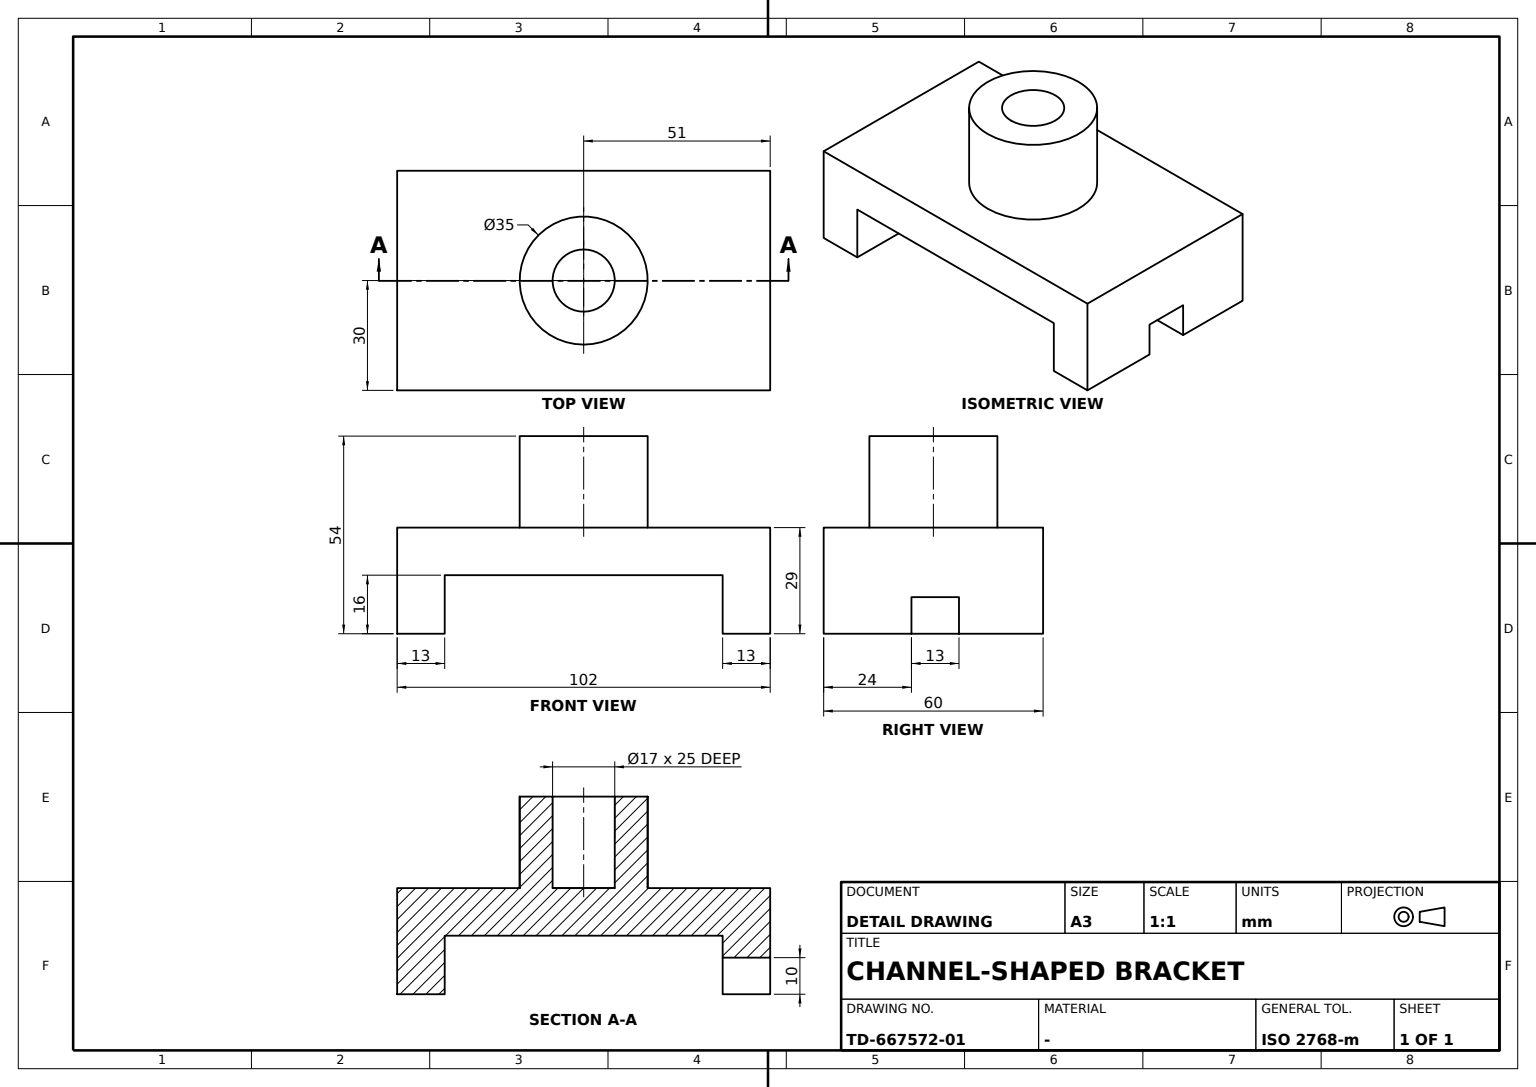
ISO-10303-21;
HEADER;
FILE_DESCRIPTION((''),'2;1');
FILE_NAME('','',(''),(''),'','','');
FILE_SCHEMA(('AUTOMOTIVE_DESIGN'));
ENDSEC;
DATA;
#1=APPLICATION_CONTEXT('');
#2=PRODUCT_CONTEXT('',#1,'mechanical');
#3=PRODUCT('','','',(#2));
#4=PRODUCT_DEFINITION_FORMATION('','',#3);
#5=PRODUCT_DEFINITION_CONTEXT('',#1,'design');
#6=PRODUCT_DEFINITION('','',#4,#5);
#7=PRODUCT_DEFINITION_SHAPE('','',#6);
#8=(LENGTH_UNIT()NAMED_UNIT(*)SI_UNIT(.MILLI.,.METRE.));
#9=(NAMED_UNIT(*)PLANE_ANGLE_UNIT()SI_UNIT($,.RADIAN.));
#10=(NAMED_UNIT(*)SI_UNIT($,.STERADIAN.)SOLID_ANGLE_UNIT());
#11=UNCERTAINTY_MEASURE_WITH_UNIT(LENGTH_MEASURE(0.005),#8,'distance_accuracy_value','');
#12=(GEOMETRIC_REPRESENTATION_CONTEXT(3)GLOBAL_UNCERTAINTY_ASSIGNED_CONTEXT((#11))GLOBAL_UNIT_ASSIGNED_CONTEXT((#8,#9,#10))REPRESENTATION_CONTEXT('',''));
#13=CARTESIAN_POINT('',(0.,38.,-29.));
#14=VERTEX_POINT('',#13);
#15=CARTESIAN_POINT('',(0.,38.,-13.));
#16=VERTEX_POINT('',#15);
#17=DIRECTION('',(0.,0.,1.));
#18=VECTOR('',#17,1000.);
#19=LINE('',#13,#18);
#20=EDGE_CURVE('',#14,#16,#19,.T.);
#21=ORIENTED_EDGE('',*,*,#20,.T.);
#22=CARTESIAN_POINT('',(-60.,38.,-13.));
#23=VERTEX_POINT('',#22);
#24=DIRECTION('',(-1.,0.,0.));
#25=VECTOR('',#24,1000.);
#26=LINE('',#15,#25);
#27=EDGE_CURVE('',#16,#23,#26,.T.);
#28=ORIENTED_EDGE('',*,*,#27,.T.);
#29=CARTESIAN_POINT('',(-60.,38.,-29.));
#30=VERTEX_POINT('',#29);
#31=LINE('',#29,#18);
#32=EDGE_CURVE('',#30,#23,#31,.T.);
#33=ORIENTED_EDGE('',*,*,#32,.F.);
#34=CARTESIAN_POINT('',(-37.,38.,-29.));
#35=VERTEX_POINT('',#34);
#36=LINE('',#13,#25);
#37=EDGE_CURVE('',#35,#30,#36,.T.);
#38=ORIENTED_EDGE('',*,*,#37,.F.);
#39=CARTESIAN_POINT('',(-37.,38.,-19.));
#40=VERTEX_POINT('',#39);
#41=DIRECTION('',(0.,0.,-1.));
#42=VECTOR('',#41,1000.);
#43=LINE('',#34,#42);
#44=EDGE_CURVE('',#40,#35,#43,.T.);
#45=ORIENTED_EDGE('',*,*,#44,.F.);
#46=CARTESIAN_POINT('',(-24.,38.,-19.));
#47=VERTEX_POINT('',#46);
#48=CARTESIAN_POINT('',(0.,38.,-19.));
#49=LINE('',#48,#25);
#50=EDGE_CURVE('',#47,#40,#49,.T.);
#51=ORIENTED_EDGE('',*,*,#50,.F.);
#52=CARTESIAN_POINT('',(-24.,38.,-29.));
#53=VERTEX_POINT('',#52);
#54=LINE('',#52,#18);
#55=EDGE_CURVE('',#53,#47,#54,.T.);
#56=ORIENTED_EDGE('',*,*,#55,.F.);
#57=EDGE_CURVE('',#14,#53,#36,.T.);
#58=ORIENTED_EDGE('',*,*,#57,.F.);
#59=EDGE_LOOP('',(#21,#28,#33,#38,#45,#51,#56,#58));
#60=FACE_BOUND('',#59,.T.);
#61=DIRECTION('',(0.,-1.,0.));
#62=AXIS2_PLACEMENT_3D('',#13,#61,#17);
#63=PLANE('',#62);
#64=ADVANCED_FACE('',(#60),#63,.T.);
#65=CARTESIAN_POINT('',(-37.,51.,-29.));
#66=VERTEX_POINT('',#65);
#67=CARTESIAN_POINT('',(-60.,51.,-29.));
#68=VERTEX_POINT('',#67);
#69=CARTESIAN_POINT('',(0.,51.,-29.));
#70=LINE('',#69,#25);
#71=EDGE_CURVE('',#66,#68,#70,.T.);
#72=ORIENTED_EDGE('',*,*,#71,.F.);
#73=VECTOR('',#61,1000.);
#74=LINE('',#65,#73);
#75=EDGE_CURVE('',#66,#35,#74,.T.);
#76=ORIENTED_EDGE('',*,*,#75,.T.);
#77=ORIENTED_EDGE('',*,*,#37,.T.);
#78=CARTESIAN_POINT('',(-60.,-38.,-29.));
#79=LINE('',#78,#73);
#80=EDGE_CURVE('',#68,#30,#79,.T.);
#81=ORIENTED_EDGE('',*,*,#80,.F.);
#82=EDGE_LOOP('',(#72,#76,#77,#81));
#83=FACE_BOUND('',#82,.T.);
#84=CARTESIAN_POINT('',(0.,-38.,-29.));
#85=AXIS2_PLACEMENT_3D('',#84,#41,#61);
#86=PLANE('',#85);
#87=ADVANCED_FACE('',(#83),#86,.T.);
#88=ORIENTED_EDGE('',*,*,#57,.T.);
#89=CARTESIAN_POINT('',(-24.,51.,-29.));
#90=VERTEX_POINT('',#89);
#91=CARTESIAN_POINT('',(-24.,-38.,-29.));
#92=LINE('',#91,#73);
#93=EDGE_CURVE('',#90,#53,#92,.T.);
#94=ORIENTED_EDGE('',*,*,#93,.F.);
#95=VERTEX_POINT('',#69);
#96=EDGE_CURVE('',#95,#90,#70,.T.);
#97=ORIENTED_EDGE('',*,*,#96,.F.);
#98=LINE('',#84,#73);
#99=EDGE_CURVE('',#95,#14,#98,.T.);
#100=ORIENTED_EDGE('',*,*,#99,.T.);
#101=EDGE_LOOP('',(#88,#94,#97,#100));
#102=FACE_BOUND('',#101,.T.);
#103=ADVANCED_FACE('',(#102),#86,.T.);
#104=ORIENTED_EDGE('',*,*,#55,.T.);
#105=CARTESIAN_POINT('',(-24.,51.,-19.));
#106=VERTEX_POINT('',#105);
#107=LINE('',#105,#73);
#108=EDGE_CURVE('',#106,#47,#107,.T.);
#109=ORIENTED_EDGE('',*,*,#108,.F.);
#110=LINE('',#89,#18);
#111=EDGE_CURVE('',#90,#106,#110,.T.);
#112=ORIENTED_EDGE('',*,*,#111,.F.);
#113=ORIENTED_EDGE('',*,*,#93,.T.);
#114=EDGE_LOOP('',(#104,#109,#112,#113));
#115=FACE_BOUND('',#114,.T.);
#116=DIRECTION('',(1.,0.,0.));
#117=AXIS2_PLACEMENT_3D('',#89,#116,#17);
#118=PLANE('',#117);
#119=ADVANCED_FACE('',(#115),#118,.F.);
#120=CARTESIAN_POINT('',(-21.5,0.,0.));
#121=VERTEX_POINT('',#120);
#122=CARTESIAN_POINT('',(-30.,0.,0.));
#123=AXIS2_PLACEMENT_3D('',#122,#17,#116);
#124=CIRCLE('',#123,8.5);
#125=EDGE_CURVE('',#121,#121,#124,.T.);
#126=ORIENTED_EDGE('',*,*,#125,.F.);
#127=EDGE_LOOP('',(#126));
#128=FACE_BOUND('',#127,.T.);
#129=CARTESIAN_POINT('',(-21.5,0.,25.));
#130=VERTEX_POINT('',#129);
#131=CARTESIAN_POINT('',(-30.,0.,25.));
#132=AXIS2_PLACEMENT_3D('',#131,#17,#116);
#133=CIRCLE('',#132,8.5);
#134=EDGE_CURVE('',#130,#130,#133,.T.);
#135=ORIENTED_EDGE('',*,*,#134,.T.);
#136=EDGE_LOOP('',(#135));
#137=FACE_BOUND('',#136,.T.);
#138=CARTESIAN_POINT('',(-30.,0.,12.5));
#139=AXIS2_PLACEMENT_3D('',#138,#17,#116);
#140=CYLINDRICAL_SURFACE('',#139,8.5);
#141=ADVANCED_FACE('',(#128,#137),#140,.F.);
#142=CARTESIAN_POINT('',(0.,-51.,-29.));
#143=VERTEX_POINT('',#142);
#144=CARTESIAN_POINT('',(0.,-51.,0.));
#145=VERTEX_POINT('',#144);
#146=LINE('',#142,#18);
#147=EDGE_CURVE('',#143,#145,#146,.T.);
#148=ORIENTED_EDGE('',*,*,#147,.T.);
#149=CARTESIAN_POINT('',(-60.,-51.,0.));
#150=VERTEX_POINT('',#149);
#151=LINE('',#144,#25);
#152=EDGE_CURVE('',#145,#150,#151,.T.);
#153=ORIENTED_EDGE('',*,*,#152,.T.);
#154=CARTESIAN_POINT('',(-60.,-51.,-29.));
#155=VERTEX_POINT('',#154);
#156=LINE('',#154,#18);
#157=EDGE_CURVE('',#155,#150,#156,.T.);
#158=ORIENTED_EDGE('',*,*,#157,.F.);
#159=LINE('',#142,#25);
#160=EDGE_CURVE('',#143,#155,#159,.T.);
#161=ORIENTED_EDGE('',*,*,#160,.F.);
#162=EDGE_LOOP('',(#148,#153,#158,#161));
#163=FACE_BOUND('',#162,.T.);
#164=AXIS2_PLACEMENT_3D('',#142,#61,#17);
#165=PLANE('',#164);
#166=ADVANCED_FACE('',(#163),#165,.T.);
#167=ORIENTED_EDGE('',*,*,#125,.T.);
#168=EDGE_LOOP('',(#167));
#169=FACE_BOUND('',#168,.T.);
#170=DIRECTION('',(0.,1.,0.));
#171=AXIS2_PLACEMENT_3D('',#144,#17,#170);
#172=PLANE('',#171);
#173=ADVANCED_FACE('',(#169),#172,.T.);
#174=CARTESIAN_POINT('',(0.,51.,0.));
#175=VERTEX_POINT('',#174);
#176=LINE('',#174,#42);
#177=EDGE_CURVE('',#175,#95,#176,.T.);
#178=ORIENTED_EDGE('',*,*,#177,.T.);
#179=ORIENTED_EDGE('',*,*,#96,.T.);
#180=ORIENTED_EDGE('',*,*,#111,.T.);
#181=CARTESIAN_POINT('',(-37.,51.,-19.));
#182=VERTEX_POINT('',#181);
#183=LINE('',#105,#25);
#184=EDGE_CURVE('',#106,#182,#183,.T.);
#185=ORIENTED_EDGE('',*,*,#184,.T.);
#186=LINE('',#181,#42);
#187=EDGE_CURVE('',#182,#66,#186,.T.);
#188=ORIENTED_EDGE('',*,*,#187,.T.);
#189=ORIENTED_EDGE('',*,*,#71,.T.);
#190=CARTESIAN_POINT('',(-60.,51.,0.));
#191=VERTEX_POINT('',#190);
#192=LINE('',#190,#42);
#193=EDGE_CURVE('',#191,#68,#192,.T.);
#194=ORIENTED_EDGE('',*,*,#193,.F.);
#195=LINE('',#174,#25);
#196=EDGE_CURVE('',#175,#191,#195,.T.);
#197=ORIENTED_EDGE('',*,*,#196,.F.);
#198=EDGE_LOOP('',(#178,#179,#180,#185,#188,#189,#194,#197));
#199=FACE_BOUND('',#198,.T.);
#200=AXIS2_PLACEMENT_3D('',#174,#170,#41);
#201=PLANE('',#200);
#202=ADVANCED_FACE('',(#199),#201,.T.);
#203=ORIENTED_EDGE('',*,*,#152,.F.);
#204=VECTOR('',#170,1000.);
#205=LINE('',#144,#204);
#206=EDGE_CURVE('',#145,#175,#205,.T.);
#207=ORIENTED_EDGE('',*,*,#206,.T.);
#208=ORIENTED_EDGE('',*,*,#196,.T.);
#209=LINE('',#149,#204);
#210=EDGE_CURVE('',#150,#191,#209,.T.);
#211=ORIENTED_EDGE('',*,*,#210,.F.);
#212=EDGE_LOOP('',(#203,#207,#208,#211));
#213=FACE_BOUND('',#212,.T.);
#214=CARTESIAN_POINT('',(-12.5,0.,0.));
#215=VERTEX_POINT('',#214);
#216=CIRCLE('',#123,17.5);
#217=EDGE_CURVE('',#215,#215,#216,.T.);
#218=ORIENTED_EDGE('',*,*,#217,.F.);
#219=EDGE_LOOP('',(#218));
#220=FACE_BOUND('',#219,.T.);
#221=ADVANCED_FACE('',(#213,#220),#172,.T.);
#222=CARTESIAN_POINT('',(-60.,-38.,-13.));
#223=VERTEX_POINT('',#222);
#224=LINE('',#22,#73);
#225=EDGE_CURVE('',#23,#223,#224,.T.);
#226=ORIENTED_EDGE('',*,*,#225,.F.);
#227=ORIENTED_EDGE('',*,*,#27,.F.);
#228=CARTESIAN_POINT('',(0.,-38.,-13.));
#229=VERTEX_POINT('',#228);
#230=LINE('',#15,#73);
#231=EDGE_CURVE('',#16,#229,#230,.T.);
#232=ORIENTED_EDGE('',*,*,#231,.T.);
#233=LINE('',#228,#25);
#234=EDGE_CURVE('',#229,#223,#233,.T.);
#235=ORIENTED_EDGE('',*,*,#234,.T.);
#236=EDGE_LOOP('',(#226,#227,#232,#235));
#237=FACE_BOUND('',#236,.T.);
#238=AXIS2_PLACEMENT_3D('',#15,#41,#61);
#239=PLANE('',#238);
#240=ADVANCED_FACE('',(#237),#239,.T.);
#241=ORIENTED_EDGE('',*,*,#134,.F.);
#242=EDGE_LOOP('',(#241));
#243=FACE_BOUND('',#242,.T.);
#244=CARTESIAN_POINT('',(-12.5,0.,25.));
#245=VERTEX_POINT('',#244);
#246=CIRCLE('',#132,17.5);
#247=EDGE_CURVE('',#245,#245,#246,.T.);
#248=ORIENTED_EDGE('',*,*,#247,.T.);
#249=EDGE_LOOP('',(#248));
#250=FACE_BOUND('',#249,.T.);
#251=CARTESIAN_POINT('',(0.,0.,25.));
#252=AXIS2_PLACEMENT_3D('',#251,#17,#116);
#253=PLANE('',#252);
#254=ADVANCED_FACE('',(#243,#250),#253,.T.);
#255=ORIENTED_EDGE('',*,*,#247,.F.);
#256=EDGE_LOOP('',(#255));
#257=FACE_BOUND('',#256,.T.);
#258=ORIENTED_EDGE('',*,*,#217,.T.);
#259=EDGE_LOOP('',(#258));
#260=FACE_BOUND('',#259,.T.);
#261=CYLINDRICAL_SURFACE('',#139,17.5);
#262=ADVANCED_FACE('',(#257,#260),#261,.T.);
#263=ORIENTED_EDGE('',*,*,#20,.F.);
#264=ORIENTED_EDGE('',*,*,#99,.F.);
#265=ORIENTED_EDGE('',*,*,#177,.F.);
#266=ORIENTED_EDGE('',*,*,#206,.F.);
#267=ORIENTED_EDGE('',*,*,#147,.F.);
#268=VERTEX_POINT('',#84);
#269=EDGE_CURVE('',#268,#143,#98,.T.);
#270=ORIENTED_EDGE('',*,*,#269,.F.);
#271=LINE('',#228,#42);
#272=EDGE_CURVE('',#229,#268,#271,.T.);
#273=ORIENTED_EDGE('',*,*,#272,.F.);
#274=ORIENTED_EDGE('',*,*,#231,.F.);
#275=EDGE_LOOP('',(#263,#264,#265,#266,#267,#270,#273,#274));
#276=FACE_BOUND('',#275,.T.);
#277=CARTESIAN_POINT('',(0.,0.,0.));
#278=AXIS2_PLACEMENT_3D('',#277,#116,#170);
#279=PLANE('',#278);
#280=ADVANCED_FACE('',(#276),#279,.T.);
#281=ORIENTED_EDGE('',*,*,#50,.T.);
#282=LINE('',#181,#73);
#283=EDGE_CURVE('',#182,#40,#282,.T.);
#284=ORIENTED_EDGE('',*,*,#283,.F.);
#285=ORIENTED_EDGE('',*,*,#184,.F.);
#286=ORIENTED_EDGE('',*,*,#108,.T.);
#287=EDGE_LOOP('',(#281,#284,#285,#286));
#288=FACE_BOUND('',#287,.T.);
#289=AXIS2_PLACEMENT_3D('',#105,#17,#24);
#290=PLANE('',#289);
#291=ADVANCED_FACE('',(#288),#290,.F.);
#292=VERTEX_POINT('',#78);
#293=LINE('',#84,#25);
#294=EDGE_CURVE('',#268,#292,#293,.T.);
#295=ORIENTED_EDGE('',*,*,#294,.T.);
#296=LINE('',#222,#42);
#297=EDGE_CURVE('',#223,#292,#296,.T.);
#298=ORIENTED_EDGE('',*,*,#297,.F.);
#299=ORIENTED_EDGE('',*,*,#234,.F.);
#300=ORIENTED_EDGE('',*,*,#272,.T.);
#301=EDGE_LOOP('',(#295,#298,#299,#300));
#302=FACE_BOUND('',#301,.T.);
#303=AXIS2_PLACEMENT_3D('',#228,#170,#41);
#304=PLANE('',#303);
#305=ADVANCED_FACE('',(#302),#304,.T.);
#306=ORIENTED_EDGE('',*,*,#294,.F.);
#307=ORIENTED_EDGE('',*,*,#269,.T.);
#308=ORIENTED_EDGE('',*,*,#160,.T.);
#309=EDGE_CURVE('',#292,#155,#79,.T.);
#310=ORIENTED_EDGE('',*,*,#309,.F.);
#311=EDGE_LOOP('',(#306,#307,#308,#310));
#312=FACE_BOUND('',#311,.T.);
#313=ADVANCED_FACE('',(#312),#86,.T.);
#314=ORIENTED_EDGE('',*,*,#283,.T.);
#315=ORIENTED_EDGE('',*,*,#44,.T.);
#316=ORIENTED_EDGE('',*,*,#75,.F.);
#317=ORIENTED_EDGE('',*,*,#187,.F.);
#318=EDGE_LOOP('',(#314,#315,#316,#317));
#319=FACE_BOUND('',#318,.T.);
#320=AXIS2_PLACEMENT_3D('',#181,#24,#41);
#321=PLANE('',#320);
#322=ADVANCED_FACE('',(#319),#321,.F.);
#323=ORIENTED_EDGE('',*,*,#297,.T.);
#324=ORIENTED_EDGE('',*,*,#309,.T.);
#325=ORIENTED_EDGE('',*,*,#157,.T.);
#326=ORIENTED_EDGE('',*,*,#210,.T.);
#327=ORIENTED_EDGE('',*,*,#193,.T.);
#328=ORIENTED_EDGE('',*,*,#80,.T.);
#329=ORIENTED_EDGE('',*,*,#32,.T.);
#330=ORIENTED_EDGE('',*,*,#225,.T.);
#331=EDGE_LOOP('',(#323,#324,#325,#326,#327,#328,#329,#330));
#332=FACE_BOUND('',#331,.T.);
#333=CARTESIAN_POINT('',(-60.,0.,0.));
#334=AXIS2_PLACEMENT_3D('',#333,#116,#170);
#335=PLANE('',#334);
#336=ADVANCED_FACE('',(#332),#335,.F.);
#337=CLOSED_SHELL('',(#64,#87,#103,#119,#141,#166,#173,#202,#221,#240,#254,#262,#280,#291,#305,#313,#322,#336));
#338=MANIFOLD_SOLID_BREP('',#337);
#339=ADVANCED_BREP_SHAPE_REPRESENTATION('',(#338),#12);
#340=SHAPE_DEFINITION_REPRESENTATION(#7,#339);
ENDSEC;
END-ISO-10303-21;
